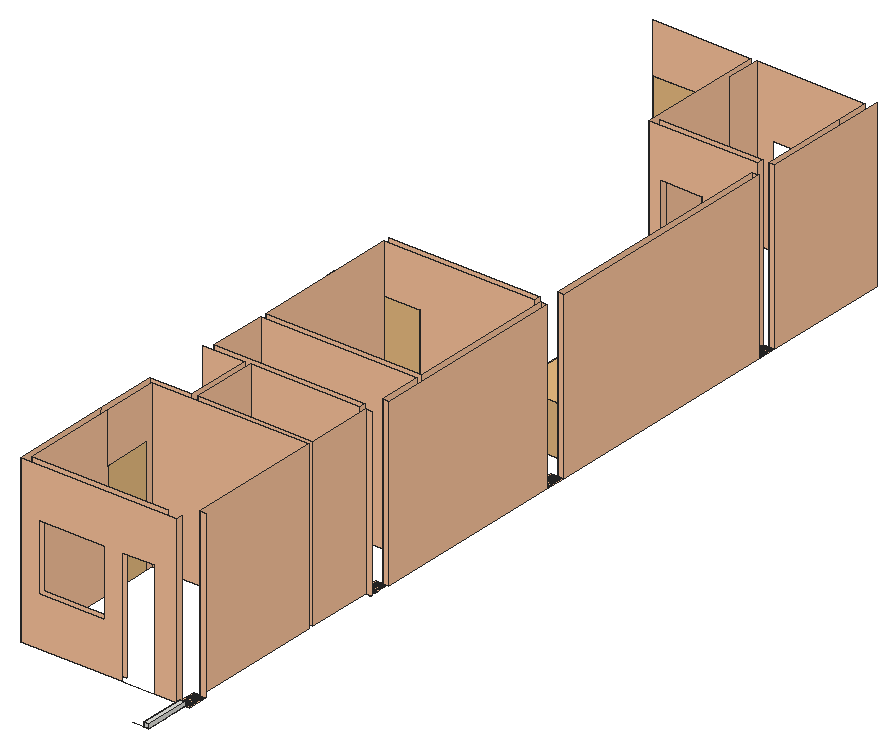
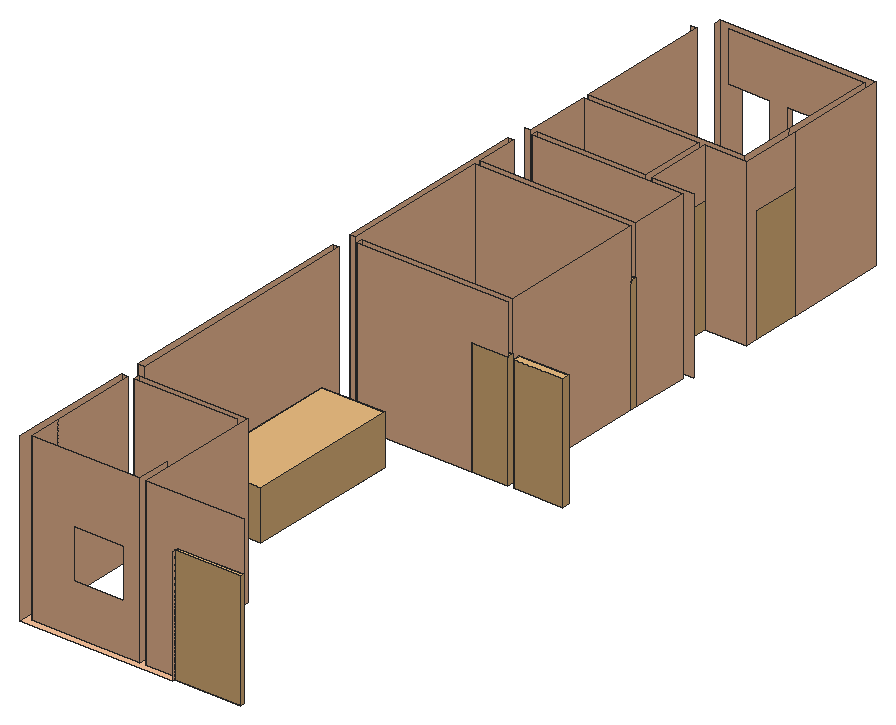
# SketchUp Ruby script. Lengths in inches.
U = 1.inch
M = Sketchup.active_model
def pt(a) = Geom::Point3d.new(a.map { |v| v * U })
def face(e, loops, mat)
  f = e.add_face(loops[0].map { |a| pt(a) })
  loops[1..].each { |l| e.add_face(l.map { |a| pt(a) }).erase! }
  f.material = f.back_material = mat if mat
  f
end
# faces: each face lists its corners as indices into pts; further lists are holes
def faces(e, pts, list, mat = nil) = list.each { |f| face(e, (f[0].is_a?(Array) ? f : [f]).map { |l| l.map { |i| pts[i] } }, mat) }
# xy, xz, yz: faces in a plane at the given z, y or x. An outline is a flat list of corners, or four numbers for a rectangle; further outlines are holes
def ring(l) = l.size == 4 ? [[l[0], l[1]], [l[2], l[1]], [l[2], l[3]], [l[0], l[3]]] : l.each_slice(2).to_a
def flat(e, list, mat, &to3) = list.each { |f| face(e, (f[0].is_a?(Array) ? f : [f]).map { |l| ring(l).map { |u, v| to3.(u, v) } }, mat) }
def xy(e, z, list, mat = nil) = flat(e, list, mat) { |x, y| [x, y, z] }
def xz(e, y, list, mat = nil) = flat(e, list, mat) { |x, z| [x, y, z] }
def yz(e, x, list, mat = nil) = flat(e, list, mat) { |y, z| [x, y, z] }
def lines(e, pts, list) = list.each { |a, b| e.add_line(pt(pts[a]), pt(pts[b])) }
# prism: a flat outline (further loops are holes) pulled along v
def prism(e, loops, v, mat = nil)
  f = face(e, loops, mat); d = Geom::Vector3d.new(v.map { |x| x * U })
  f.pushpull(f.normal.samedirection?(d) ? d.length : -d.length)
end
def box(e, o, s, mat = nil) = prism(e, [[o, [o[0] + s[0], o[1], o[2]], [o[0] + s[0], o[1] + s[1], o[2]], [o[0], o[1] + s[1], o[2]]]], [0, 0, s[2]], mat)
def at(x, y, z, deg = 0) = Geom::Transformation.translation(pt([x, y, z])) * Geom::Transformation.rotation(ORIGIN, Z_AXIS, deg.degrees)
def axes(o, x, y, z) = Geom::Transformation.new([*x, 0, *y, 0, *z, 0, *pt(o).to_a, 1])
def part(name) = M.definitions.add(name)
# library, detail: a bought-in or finely detailed component or shape, given as its bounding box
def library(name, o, s) = part(name).tap { |d| box(d.entities, o, s) }
def detail(e, o, s) = box(e.add_group.entities, o, s)
def put(e, d, t, mat = nil) = e.add_instance(d, t).tap { |i| i.material = mat if mat }
def group(e, t, mat = nil) = e.add_group.tap { |g| g.transformation = t; g.material = mat if mat }.entities
root = M.entities
M.materials.add("[Color A01]2").color = [255, 204, 204]
M.materials.add("[Color A02]1").color = [252, 197, 157]
c1 = library("Group\#55",[0,0,0],[42.67,2.97,87.375])
c2 = library("Group\#37",[0,0,0],[42.67,2.97,87.375])
c3 = library("Group\#46",[0,0,0],[42.67,2.97,87.375])
c4 = library("Sliding door\#1",[32.62,66.51,0],[146.81,8.35,98.97])
c5 = library("Sofa 005",[-44.88,-17.99,0],[89.76,35.98,35.98])
box(root,[168.96,13.0625,131.89],[3.93,33,3])
xy(root,131.89,[[150.53,46.0625,166.9,50.62],[166.9,46.0625,175.89,46.0625,175.89,61,171.33,61,171.33,60.12,174.88,60.12,174.88,47.08,167.91,47.08,167.91,50.62,166.9,50.62],[167.91,47.08,168.17,47.08,168.54,47.46,167.91,48.09],[168.17,47.08,168.93,47.08,168.54,47.46],[168.93,47.08,169.94,47.08,170.32,47.46,169.42,48.35,168.54,47.46],
  [169.94,47.08,170.7,47.08,170.32,47.46],[170.7,47.08,171.71,47.08,172.09,47.46,171.19,48.36,170.32,47.46],[171.71,47.08,172.47,47.08,172.09,47.46],[172.47,47.08,173.49,47.08,173.85,47.47,172.95,48.37,172.09,47.46],[173.49,47.08,174.25,47.08,173.85,47.47],
  [174.25,47.08,174.88,47.08,174.88,48.22,174.7,48.4,173.85,47.47],[168.54,47.46,169.42,48.35,168.54,49.23,167.91,48.6,167.91,48.09],[170.32,47.46,171.19,48.36,170.3,49.25,169.42,48.35],[172.09,47.46,172.95,48.37,172.07,49.26,171.19,48.36],[173.85,47.47,174.7,48.4,173.82,49.27,172.95,48.37],
  [174.88,48.22,174.88,48.6,174.7,48.4],[169.42,48.35,170.3,49.25,169.42,50.13,168.54,49.23],[171.19,48.36,172.07,49.26,171.18,50.14,170.3,49.25],[172.95,48.37,173.82,49.27,172.94,50.15,172.07,49.26],[174.7,48.4,174.88,48.6,174.88,49.99,174.69,50.17,173.82,49.27],
  [167.91,48.6,168.54,49.23,167.91,49.86],[168.54,49.23,169.42,50.13,168.93,50.62,168.16,50.62,167.91,50.37,167.91,49.86],[170.3,49.25,171.18,50.14,170.7,50.62,169.9,50.62,169.42,50.13],[172.07,49.26,172.94,50.15,172.06,51.04,171.18,50.14],[173.82,49.27,174.69,50.17,173.82,51.05,172.94,50.15],
  [174.88,49.99,174.88,50.37,174.69,50.17],[169.42,50.13,169.9,50.62,168.93,50.62],[171.18,50.14,172.06,51.04,171.33,51.76,171.33,50.62,170.7,50.62],[172.94,50.15,173.82,51.05,172.93,51.93,172.06,51.04],[174.69,50.17,174.88,50.37,174.88,51.76,174.69,51.95,173.82,51.05],
  [167.91,50.37,168.16,50.62,167.91,50.62],[166.9,50.62,167.91,50.62,167.91,60.12,171.33,60.12,171.33,61.13,166.9,61.13],[167.91,50.62,168.16,50.62,168.54,51.01,167.91,51.63],[168.16,50.62,168.93,50.62,168.54,51.01],[168.93,50.62,169.9,50.62,170.3,51.02,169.42,51.9,168.54,51.01],
  [169.9,50.62,170.7,50.62,170.3,51.02],[170.7,50.62,171.33,50.62,171.33,51.76,171.18,51.92,170.3,51.02],[168.54,51.01,169.42,51.9,168.54,52.78,167.91,52.14,167.91,51.63],[170.3,51.02,171.18,51.92,170.3,52.8,169.42,51.9],[172.06,51.04,172.93,51.93,172.06,52.8125,171.33,52.08,171.33,51.76],
  [173.82,51.05,174.69,51.95,173.8125,52.83,172.93,51.93],[171.33,51.76,171.33,52.08,171.18,51.92],[174.88,51.76,174.88,52.14,174.69,51.95],[169.42,51.9,170.3,52.8,169.42,53.67,168.54,52.78],[171.18,51.92,171.33,52.08,171.33,53.53,171.18,53.69,170.3,52.8],
  [172.93,51.93,173.8125,52.83,172.93,53.71,172.06,52.8125],[174.69,51.95,174.88,52.14,174.88,53.53,174.69,53.72,173.8125,52.83],[171.33,52.08,172.06,52.8125,171.33,53.53],[167.91,52.14,168.54,52.78,167.91,53.41],[168.54,52.78,169.42,53.67,168.55,54.55,167.91,53.91,167.91,53.41],
  [170.3,52.8,171.18,53.69,170.3,54.57,169.42,53.67],[172.06,52.8125,172.93,53.71,172.06,54.58,171.33,53.85,171.33,53.53],[173.8125,52.83,174.69,53.72,173.8125,54.6,172.93,53.71],[171.33,53.53,171.33,53.85,171.18,53.69],[174.88,53.53,174.88,53.91,174.69,53.72],
  [169.42,53.67,170.3,54.57,169.43,55.43,168.55,54.55],[171.18,53.69,171.33,53.85,171.33,55.31,171.18,55.46,170.3,54.57],[172.93,53.71,173.8125,54.6,172.93,55.48,172.06,54.58],[171.33,53.85,172.06,54.58,171.33,55.31],[167.91,53.91,168.55,54.55,167.91,55.18],
  [168.55,54.55,169.43,55.43,168.55,56.32,167.91,55.6875,167.91,55.18],[170.3,54.57,171.18,55.46,170.32,56.32,169.43,55.43],[172.06,54.58,172.93,55.48,172.06,56.36,171.33,55.62,171.33,55.31],[173.8125,54.6,174.69,55.49,173.8125,56.37,172.93,55.48],[171.33,55.31,171.33,55.62,171.18,55.46],
  [169.43,55.43,170.32,56.32,169.43,57.21,168.55,56.32],[171.18,55.46,171.33,55.62,171.33,57.08,171.21,57.21,170.32,56.32],[172.93,55.48,173.8125,56.37,172.93,57.25,172.06,56.36],[174.69,55.49,174.88,55.6875,174.88,57.08,174.69,57.27,173.8125,56.37],[171.33,55.62,172.06,56.36,171.33,57.08],
  [167.91,55.6875,168.55,56.32,167.91,56.95],[168.55,56.32,169.43,57.21,168.55,58.09,167.91,57.46,167.91,56.95],[170.32,56.32,171.21,57.21,170.32,58.09,169.43,57.21],[172.06,56.36,172.93,57.25,172.09,58.09,171.33,57.33,171.33,57.08],[173.8125,56.37,174.69,57.27,173.8125,58.15,172.93,57.25],
  [171.33,57.08,171.33,57.33,171.21,57.21],[174.88,57.08,174.88,57.46,174.69,57.27],[169.43,57.21,170.32,58.09,169.43,58.98,168.55,58.09],[171.21,57.21,171.33,57.33,171.33,58.85,171.21,58.98,170.32,58.09],[172.93,57.25,173.8125,58.15,172.98,58.98,172.09,58.09],
  [174.69,57.27,174.88,57.46,174.88,58.85,174.69,59.04,173.8125,58.15],[171.33,57.33,172.09,58.09,171.33,58.85],[168.55,58.09,169.43,58.98,168.55,59.86,167.91,59.23,167.91,58.73],[170.32,58.09,171.21,58.98,170.32,59.86,169.43,58.98],[172.09,58.09,172.98,58.98,172.09,59.86,171.33,59.11,171.33,58.85],
  [173.8125,58.15,174.69,59.04,173.87,59.86,172.98,58.98],[171.33,58.85,171.33,59.11,171.21,58.98],[174.88,58.85,174.88,59.23,174.69,59.04],[169.43,58.98,170.32,59.86,170.07,60.12,168.8,60.12,168.55,59.86],[171.21,58.98,171.33,59.11,171.33,60.12,170.57,60.12,170.32,59.86],
  [172.98,58.98,173.87,59.86,173.61,60.12,172.35,60.12,172.09,59.86],[174.69,59.04,174.88,59.23,174.88,60.12,174.12,60.12,173.87,59.86],[171.33,59.11,172.09,59.86,171.84,60.12,171.33,60.12],[167.91,59.23,168.55,59.86,168.29,60.12,167.91,60.12],[168.55,59.86,168.8,60.12,168.29,60.12],
  [170.32,59.86,170.57,60.12,170.07,60.12],[172.09,59.86,172.35,60.12,171.84,60.12],[173.87,59.86,174.12,60.12,173.61,60.12],[166.89,212.2,166.9,216.63],[171.33,212.2,175.89,212.21],
  [167.91,213.21,168.17,213.21,168.55,213.59,167.91,214.22],[168.93,213.21,169.94,213.21,170.32,213.59,169.43,214.48,168.55,213.59],[169.94,213.21,170.7,213.21,170.32,213.59],[170.7,213.21,171.71,213.21,172.09,213.59,171.21,214.48,170.32,213.59],[171.71,213.21,172.47,213.21,172.09,213.59],
  [172.47,213.21,173.49,213.21,173.87,213.59,172.98,214.48,172.09,213.59],[173.49,213.21,174.25,213.21,173.87,213.59],[174.25,213.21,174.88,213.21,174.88,214.22,174.69,214.42,173.87,213.59],[168.55,213.59,169.43,214.48,168.55,215.36,167.91,214.73,167.91,214.22],[170.32,213.59,171.21,214.48,170.32,215.36,169.43,214.48],
  [172.09,213.59,172.98,214.48,172.09,215.36,171.21,214.48],[173.87,213.59,174.69,214.42,173.8125,215.3125,172.98,214.48],[169.43,214.48,170.32,215.36,169.43,216.25,168.55,215.36],[171.21,214.48,172.09,215.36,171.21,216.25,170.32,215.36],[172.98,214.48,173.8125,215.3125,172.93,216.21,172.09,215.36],
  [167.91,214.73,168.55,215.36,167.91,216],[173.8125,215.3125,174.69,216.1875,173.8125,217.08,172.93,216.21],[168.55,215.36,169.43,216.25,169.05,216.63,168.04,216.63,167.91,216.5,167.91,216],[170.32,215.36,171.21,216.25,170.83,216.63,169.8125,216.63,169.43,216.25],[172.09,215.36,172.93,216.21,172.06,217.1,171.21,216.25],
  [174.88,216,174.88,216.38,174.69,216.1875],[174.69,216.1875,174.88,216.38,174.88,217.77,174.6875,217.96,173.8125,217.08],[172.93,216.21,173.8125,217.08,172.93,217.98,172.06,217.1],[169.43,216.25,169.8125,216.63,169.05,216.63],[171.21,216.25,172.06,217.1,171.33,217.83,171.33,216.63,170.83,216.63],
  [167.91,216.5,168.04,216.63,167.91,216.63],[166.9,216.63,167.91,216.63,167.91,226.13,171.33,226.13,171.33,227.14,166.9,227.14],[167.91,216.63,168.04,216.63,168.55,217.14,167.91,217.77],[169.05,216.63,169.8125,216.63,170.32,217.14,169.43,218.02,168.55,217.14],[169.8125,216.63,170.83,216.63,170.32,217.14],
  [170.83,216.63,171.33,216.63,171.33,217.83,171.18,217.99,170.32,217.14],[173.8125,217.08,174.6875,217.96,173.8,218.85,172.93,217.98],[172.06,217.1,172.93,217.98,172.06,218.87,171.33,218.15,171.33,217.83],[168.55,217.14,169.43,218.02,168.55,218.91,167.91,218.28,167.91,217.77],[170.32,217.14,171.18,217.99,170.3,218.89,169.43,218.02],
  [174.88,217.77,174.88,218.15,174.6875,217.96],[171.33,217.83,171.33,218.15,171.18,217.99],[174.6875,217.96,174.88,218.15,174.88,219.54,174.6875,219.73,173.8,218.85],[172.93,217.98,173.8,218.85,172.92,219.73,172.06,218.87],[171.18,217.99,171.33,218.15,171.33,219.61,171.18,219.77,170.3,218.89],
  [171.33,218.15,172.06,218.87,171.33,219.61],[167.91,218.28,168.55,218.91,167.91,219.54],[173.8,218.85,174.6875,219.73,173.8,220.62,172.92,219.73],[172.06,218.87,172.92,219.73,172.03,220.62,171.33,219.92,171.33,219.61],[170.3,218.89,171.18,219.77,170.3,220.66,169.42,219.78],
  [174.88,219.54,174.88,219.92,174.6875,219.73],[171.33,219.61,171.33,219.92,171.18,219.77],[174.6875,219.73,174.88,219.92,174.88,221.32,174.6875,221.51,173.8,220.62],[171.18,219.77,171.33,219.92,171.33,221.32,171.14,221.51,170.3,220.66],[171.33,219.92,172.03,220.62,171.33,221.32],
  [172.03,220.62,172.92,221.51,172.03,222.39,171.33,221.7,171.33,221.32],[173.8,220.62,174.6875,221.51,173.8,222.39,172.92,221.51],[170.3,220.66,171.14,221.51,170.28,222.37,169.44,221.54],[171.33,221.32,171.33,221.7,171.14,221.51],[174.88,221.32,174.88,221.7,174.6875,221.51],
  [171.14,221.51,171.33,221.7,171.33,223.09,171.18,223.25,170.28,222.37],[172.92,221.51,173.8,222.39,172.92,223.28,172.03,222.39],[174.6875,221.51,174.88,221.7,174.88,223.09,174.6875,223.28,173.8,222.39],[169.44,221.54,170.28,222.37,169.39,223.26,168.55,222.44],[171.33,221.7,172.03,222.39,171.33,223.09],
  [167.91,221.82,168.55,222.44,167.91,223.09],[173.8,222.39,174.6875,223.28,173.8,224.16,172.92,223.28],[171.33,223.09,171.33,223.4,171.18,223.25],[174.88,223.09,174.88,223.47,174.6875,223.28],[171.18,223.25,171.33,223.4,171.33,224.86,171.19,225,170.29,224.13],
  [169.39,223.26,170.29,224.13,169.41,225.02,168.5,224.15],[172.92,223.28,173.8,224.16,172.97,225,172.07,224.12],[174.6875,223.28,174.88,223.47,174.88,224.86,174.6875,225.05,173.8,224.16],[167.91,223.6,168.5,224.15,167.91,224.73],[172.07,224.12,172.97,225,172.09,225.88,171.33,225.14,171.33,224.86],
  [168.5,224.15,169.41,225.02,168.53,225.89,167.91,225.37,167.91,224.73],[173.8,224.16,174.6875,225.05,173.86,225.875,172.97,225],[171.33,224.86,171.33,225.14,171.19,225],[174.88,224.86,174.88,225.24,174.6875,225.05],[171.19,225,171.33,225.14,171.33,226.13,170.57,226.13,170.3125,225.88],
  [169.41,225.02,170.3125,225.88,170.07,226.13,168.8,226.13,168.53,225.89],[173.86,225.875,174.12,226.13,173.61,226.13],[170.3125,225.88,170.57,226.13,170.07,226.13],[172.09,225.88,172.35,226.13,171.84,226.13],[168.53,225.89,168.8,226.13,168.29,226.13],
  [171.33,227.14,171.33,258.67,77.375,258.67,77.375,263.23,171.33,263.23,171.33,371.25,175.89,371.25,175.89,227.14],[83.33,371.24,166.9,375.68],[166.9,371.24,171.33,371.24,171.33,371.25,175.89,371.25,175.89,386.1875,171.33,386.1875,171.33,385.3,174.88,385.3,174.88,372.26,167.91,372.26,167.91,375.68,166.9,375.68],[167.91,372.26,168.17,372.26,168.55,372.64,167.91,373.27],[168.17,372.26,168.93,372.26,168.55,372.64],
  [168.93,372.26,169.94,372.26,170.32,372.64,169.43,373.52,168.55,372.64],[169.94,372.26,170.7,372.26,170.32,372.64],[170.7,372.26,171.71,372.26,172.09,372.64,171.21,373.52,170.32,372.64],[171.71,372.26,172.47,372.26,172.09,372.64],[172.47,372.26,173.49,372.26,173.87,372.64,172.98,373.52,172.09,372.64],
  [173.49,372.26,174.25,372.26,173.87,372.64],[174.25,372.26,174.88,372.26,174.88,373.27,174.69,373.46,173.87,372.64],[168.55,372.64,169.43,373.52,168.55,374.41,167.91,373.78,167.91,373.27],[170.32,372.64,171.21,373.52,170.32,374.41,169.43,373.52],[172.09,372.64,172.98,373.52,172.09,374.41,171.21,373.52],
  [173.87,372.64,174.69,373.46,173.8125,374.36,172.98,373.52],[174.88,373.27,174.88,373.65,174.69,373.46],[174.69,373.46,174.88,373.65,174.88,375.04,174.69,375.23,173.8125,374.36],[169.43,373.52,170.32,374.41,169.43,375.3,168.55,374.41],[171.21,373.52,172.09,374.41,171.21,375.3,170.32,374.41],
  [172.98,373.52,173.8125,374.36,172.93,375.25,172.09,374.41],[167.91,373.78,168.55,374.41,167.91,375.04],[173.8125,374.36,174.69,375.23,173.8125,376.13,172.93,375.25],[168.55,374.41,169.43,375.3,169.05,375.68,168.04,375.68,167.91,375.55,167.91,375.04],[170.32,374.41,171.21,375.3,170.83,375.68,169.8125,375.68,169.43,375.3],
  [172.09,374.41,172.93,375.25,172.06,376.14,171.21,375.3],[174.88,375.04,174.88,375.42,174.69,375.23],[174.69,375.23,174.88,375.42,174.88,376.82,174.69,377.01,173.8125,376.13],[172.93,375.25,173.8125,376.13,172.93,377.02,172.06,376.14],[169.43,375.3,169.8125,375.68,169.05,375.68],
  [171.21,375.3,172.06,376.14,171.33,376.88,171.33,375.68,170.83,375.68],[167.91,375.55,168.04,375.68,167.91,375.68],[166.9,375.68,167.91,375.68,167.91,385.3,171.33,385.3,171.33,386.1875,166.9,386.1875],[167.91,375.68,168.04,375.68,168.55,376.18,167.91,376.82],[168.04,375.68,169.05,375.68,168.55,376.18],
  [169.05,375.68,169.8125,375.68,170.32,376.18,169.43,377.07,168.55,376.18],[169.8125,375.68,170.83,375.68,170.32,376.18],[170.83,375.68,171.33,375.68,171.33,376.88,171.18,377.04,170.32,376.18],[173.8125,376.13,174.69,377.01,173.8125,377.9,172.93,377.02],[172.06,376.14,172.93,377.02,172.06,377.92,171.33,377.19,171.33,376.88],
  [168.55,376.18,169.43,377.07,168.55,377.95,167.91,377.32,167.91,376.82],[170.32,376.18,171.18,377.04,170.3,377.93,169.43,377.07],[174.88,376.82,174.88,377.19,174.69,377.01],[171.33,376.88,171.33,377.19,171.18,377.04],[174.69,377.01,174.88,377.19,174.88,378.59,174.69,378.78,173.8125,377.9],
  [172.93,377.02,173.8125,377.9,172.93,378.8,172.06,377.92],[171.18,377.04,171.33,377.19,171.33,378.65,171.18,378.8125,170.3,377.93],[169.43,377.07,170.3,377.93,169.42,378.83,168.55,377.95],[171.33,377.19,172.06,377.92,171.33,378.65],[167.91,377.32,168.55,377.95,167.91,378.59],
  [173.8125,377.9,174.69,378.78,173.8125,379.67,172.93,378.8],[172.06,377.92,172.93,378.8,172.06,379.69,171.33,378.97,171.33,378.65],[170.3,377.93,171.18,378.8125,170.3,379.71,169.42,378.83],[168.55,377.95,169.42,378.83,168.54,379.72,167.91,379.09,167.91,378.59],[174.88,378.59,174.88,378.97,174.69,378.78],
  [171.33,378.65,171.33,378.97,171.18,378.8125],[174.69,378.78,174.88,378.97,174.88,380.36,174.69,380.55,173.8125,379.67],[172.93,378.8,173.8125,379.67,172.93,380.57,172.06,379.69],[171.18,378.8125,171.33,378.97,171.33,380.43,171.18,380.58,170.3,379.71],[169.42,378.83,170.3,379.71,169.42,380.6,168.54,379.72],
  [171.33,378.97,172.06,379.69,171.33,380.43],[167.91,379.09,168.54,379.72,167.91,380.36],[173.8125,379.67,174.69,380.55,173.82,381.45,172.93,380.57],[172.06,379.69,172.93,380.57,172.06,381.46,171.33,380.74,171.33,380.43],[170.3,379.71,171.18,380.58,170.3,381.48,169.42,380.6],
  [168.54,379.72,169.42,380.6,168.54,381.49,167.91,380.87,167.91,380.36],[174.88,380.36,174.88,380.74,174.69,380.55],[171.33,380.43,171.33,380.74,171.18,380.58],[174.69,380.55,174.88,380.74,174.88,382.13,174.69,382.33,173.82,381.45],[172.93,380.57,173.82,381.45,172.94,382.35,172.06,381.46],
  [171.18,380.58,171.33,380.74,171.33,382.2,171.18,382.36,170.3,381.48],[169.42,380.6,170.3,381.48,169.42,382.37,168.54,381.49],[171.33,380.74,172.06,381.46,171.33,382.2],[167.91,380.87,168.54,381.49,167.91,382.13],[173.82,381.45,174.69,382.33,173.82,383.23,172.94,382.35],
  [172.06,381.46,172.94,382.35,172.07,383.25,171.33,382.51,171.33,382.2],[170.3,381.48,171.18,382.36,170.3,383.25,169.42,382.37],[168.54,381.49,169.42,382.37,168.54,383.27,167.91,382.64,167.91,382.13],[174.88,382.13,174.88,382.51,174.69,382.33],[171.33,382.2,171.33,382.51,171.18,382.36],
  [174.69,382.33,174.88,382.51,174.88,383.91,174.7,384.11,173.82,383.23],[172.94,382.35,173.82,383.23,172.96,384.14,172.07,383.25],[171.18,382.36,171.33,382.51,171.33,384,171.19,384.14,170.3,383.25],[169.42,382.37,170.3,383.25,169.42,384.15,168.54,383.27],[171.33,382.51,172.07,383.25,171.33,384],
  [167.91,382.64,168.54,383.27,167.91,383.91],[173.82,383.23,174.7,384.11,173.85,385.03,172.96,384.14],[170.3,383.25,171.19,384.14,170.32,385.04,169.42,384.15],[172.07,383.25,172.96,384.14,172.09,385.04,171.33,384.29,171.33,384],[168.54,383.27,169.42,384.15,168.54,385.04,167.91,384.41,167.91,383.91],
  [174.88,383.91,174.88,384.29,174.7,384.11],[171.33,384,171.33,384.29,171.19,384.14],[174.7,384.11,174.88,384.29,174.88,385.3,174.12,385.3,173.85,385.03],[171.19,384.14,171.33,384.29,171.33,385.3,170.57,385.3,170.32,385.04],[172.96,384.14,173.85,385.03,173.61,385.3,172.35,385.3,172.09,385.04],
  [169.42,384.15,170.32,385.04,170.07,385.3,168.8,385.3,168.54,385.04],[171.33,384.29,172.09,385.04,171.84,385.3,171.33,385.3],[167.91,384.41,168.54,385.04,168.29,385.3,167.91,385.3],[173.85,385.03,174.12,385.3,173.61,385.3],[168.54,385.04,168.8,385.3,168.29,385.3],
  [170.32,385.04,170.57,385.3,170.07,385.3],[172.09,385.04,172.35,385.3,171.84,385.3],[166.9,563.34,171.33,563.34,171.33,564.35,167.91,564.35,167.91,573.85,166.9,573.85],[171.33,563.34,175.89,563.34,175.89,578.28,166.9,578.28,166.9,573.85,167.91,573.85,167.91,577.27,174.88,577.27,174.88,564.35,171.33,564.35],[167.91,564.35,168.17,564.35,168.55,564.73,167.91,565.36],
  [168.17,564.35,168.93,564.35,168.55,564.73],[168.93,564.35,169.94,564.35,170.32,564.73,169.43,565.62,168.55,564.73],[169.94,564.35,170.7,564.35,170.32,564.73],[170.7,564.35,171.33,564.35,171.33,565.49,171.21,565.62,170.32,564.73],[171.33,564.35,171.71,564.35,172.09,564.73,171.33,565.49],
  [171.71,564.35,172.47,564.35,172.09,564.73],[172.47,564.35,173.49,564.35,173.87,564.73,172.98,565.62,172.09,564.73],[173.49,564.35,174.25,564.35,173.87,564.73],[174.25,564.35,174.88,564.35,174.88,565.36,174.69,565.56,173.87,564.73],[168.55,564.73,169.43,565.62,168.55,566.5,167.91,565.87,167.91,565.36],
  [170.32,564.73,171.21,565.62,170.32,566.5,169.43,565.62],[172.09,564.73,172.98,565.62,172.09,566.5,171.33,565.74,171.33,565.49],[173.87,564.73,174.69,565.56,173.8125,566.45,172.98,565.62],[174.88,565.36,174.88,565.74,174.69,565.56],[171.33,565.49,171.33,565.74,171.21,565.62],
  [174.69,565.56,174.88,565.74,174.88,567.14,174.6875,567.33,173.8125,566.45],[169.43,565.62,170.32,566.5,169.43,567.39,168.55,566.5],[171.21,565.62,171.33,565.74,171.33,567.26,171.21,567.39,170.32,566.5],[172.98,565.62,173.8125,566.45,172.93,567.34,172.09,566.5],[171.33,565.74,172.09,566.5,171.33,567.26],
  [167.91,565.87,168.55,566.5,167.91,567.14],[173.8125,566.45,174.6875,567.33,173.8,568.21,172.93,567.34],[168.55,566.5,169.43,567.39,168.55,568.28,167.91,567.64,167.91,567.14],[170.32,566.5,171.21,567.39,170.32,568.28,169.43,567.39],[172.09,566.5,172.93,567.34,172.06,568.24,171.33,567.52,171.33,567.26],
  [174.88,567.14,174.88,567.52,174.6875,567.33],[171.33,567.26,171.33,567.52,171.21,567.39],[174.6875,567.33,174.88,567.52,174.88,568.91,174.6875,569.1,173.8,568.21],[172.93,567.34,173.8,568.21,172.92,569.1,172.06,568.24],[169.43,567.39,170.32,568.28,169.43,569.16,168.55,568.28],
  [171.21,567.39,171.33,567.52,171.33,568.97,171.18,569.13,170.32,568.28],[171.33,567.52,172.06,568.24,171.33,568.97],[167.91,567.64,168.55,568.28,167.91,568.91],[173.8,568.21,174.6875,569.1,173.8,569.99,172.92,569.1],[172.06,568.24,172.92,569.1,172.03,569.99,171.33,569.29,171.33,568.97],
  [168.55,568.28,169.43,569.16,168.55,570.05,167.91,569.42,167.91,568.91],[170.32,568.28,171.18,569.13,170.3,570.03,169.43,569.16],[174.88,568.91,174.88,569.29,174.6875,569.1],[171.33,568.97,171.33,569.29,171.18,569.13],[172.92,569.1,173.8,569.99,172.92,570.87,172.03,569.99],
  [174.6875,569.1,174.88,569.29,174.88,570.68,174.6875,570.87,173.8,569.99],[171.18,569.13,171.33,569.29,171.33,570.68,171.14,570.87,170.3,570.03],[169.43,569.16,170.3,570.03,169.42,570.92,168.55,570.05],[171.33,569.29,172.03,569.99,171.33,570.68],[167.91,569.42,168.55,570.05,167.91,570.68],
  [172.03,569.99,172.92,570.87,172.03,571.76,171.33,571.0625,171.33,570.68],[173.8,569.99,174.6875,570.87,173.8,571.76,172.92,570.87],[170.3,570.03,171.14,570.87,170.26,571.76,169.42,570.92],[168.55,570.05,169.42,570.92,168.55,571.81,167.91,571.1875,167.91,570.68],[171.33,570.68,171.33,571.0625,171.14,570.87],
  [174.88,570.68,174.88,571.0625,174.6875,570.87],[171.14,570.87,171.33,571.0625,171.33,572.46,171.14,572.65,170.26,571.76],[172.92,570.87,173.8,571.76,172.92,572.65,172.03,571.76],[174.6875,570.87,174.88,571.0625,174.88,572.46,174.6875,572.65,173.8,571.76],[169.42,570.92,170.26,571.76,169.39,572.63,168.55,571.81],
  [171.33,571.0625,172.03,571.76,171.33,572.46],[167.91,571.1875,168.55,571.81,167.91,572.46],[170.26,571.76,171.14,572.65,170.28,573.51,169.39,572.63],[172.03,571.76,172.92,572.65,172.03,573.53,171.33,572.84,171.33,572.46],[173.8,571.76,174.6875,572.65,173.8,573.53,172.92,572.65],
  [168.55,571.81,169.39,572.63,168.49,573.52,167.91,572.96,167.91,572.46],[171.33,572.46,171.33,572.84,171.14,572.65],[174.88,572.46,174.88,572.84,174.6875,572.65],[169.39,572.63,170.28,573.51,169.94,573.85,168.83,573.85,168.49,573.52],[171.14,572.65,171.33,572.84,171.33,573.85,170.63,573.85,170.28,573.51],
  [172.92,572.65,173.8,573.53,172.92,574.42,172.03,573.53],[174.6875,572.65,174.88,572.84,174.88,574.23,174.6875,574.42,173.8,573.53],[171.33,572.84,172.03,573.53,171.18,574.38,170.63,573.85,171.33,573.85],[167.91,572.96,168.49,573.52,168.17,573.85,167.91,573.85],[170.28,573.51,170.63,573.85,169.94,573.85],
  [168.49,573.52,168.83,573.85,168.17,573.85],[172.03,573.53,172.92,574.42,172.07,575.26,171.18,574.38],[173.8,573.53,174.6875,574.42,173.8,575.3,172.92,574.42],[87.89,573.85,87.89,665.91,64.84,665.91,64.84,670.34,175.89,670.34,175.89,578.28,171.33,578.28,171.33,665.91,92.44,665.91,92.44,578.28,96.37,578.28,96.37,573.85],[126.38,573.85,166.9,578.28],
  [167.91,573.85,168.17,573.85,167.91,574.1],[168.17,573.85,168.83,573.85,169.39,574.4,168.5,575.29,167.91,574.73,167.91,574.1],[168.83,573.85,169.94,573.85,169.39,574.4],[169.94,573.85,170.63,573.85,171.18,574.38,170.29,575.27,169.39,574.4],[174.88,574.23,174.88,574.61,174.6875,574.42],
  [171.18,574.38,172.07,575.26,171.19,576.14,170.29,575.27],[169.39,574.4,170.29,575.27,169.41,576.16,168.5,575.29],[172.92,574.42,173.8,575.3,172.97,576.14,172.07,575.26],[174.6875,574.42,174.88,574.61,174.88,576,174.6875,576.19,173.8,575.3],[167.91,574.73,168.5,575.29,167.91,575.875],
  [172.07,575.26,172.97,576.14,172.09,577.02,171.19,576.14],[170.29,575.27,171.19,576.14,170.3125,577.02,169.41,576.16],[168.5,575.29,169.41,576.16,168.53,577.03,167.91,576.51,167.91,575.875],[173.8,575.3,174.6875,576.19,173.86,577.02,172.97,576.14],[174.88,576,174.88,576.38,174.6875,576.19],
  [171.19,576.14,172.09,577.02,171.84,577.27,170.57,577.27,170.3125,577.02],[172.97,576.14,173.86,577.02,173.61,577.27,172.35,577.27,172.09,577.02],[169.41,576.16,170.3125,577.02,170.07,577.27,168.8,577.27,168.53,577.03],[174.6875,576.19,174.88,576.38,174.88,577.27,174.12,577.27,173.86,577.02],[167.91,576.51,168.53,577.03,168.29,577.27,167.91,577.27],
  [170.3125,577.02,170.57,577.27,170.07,577.27],[172.09,577.02,172.35,577.27,171.84,577.27],[173.86,577.02,174.12,577.27,173.61,577.27],[168.53,577.03,168.8,577.27,168.29,577.27]],"[Color A02]1")
xz(root,46.0625,[[[52.9375,131.89,126.53,131.89,126.53,215.89,150.53,215.89,150.53,131.89,166.9,131.89,166.9,251.89,52.9375,251.89],[66.6875,167.89,114.6875,215.89]]],"[Color A02]1")
xz(root,50.62,[[[57.37,131.89,57.37,251.89,156.53,251.89,156.53,215.89,126.53,215.89,126.53,131.89],[66.6875,167.89,114.6875,215.89]]],"[Color A02]1")
xz(root,61,[[171.33,131.89,175.89,251.89]],"[Color A02]1")
xz(root,119.63,[[52.9375,131.89,57.37,215.89]],"[Color A02]1")
xz(root,160.15,[[57.37,131.89,171.33,251.89]],"[Color A02]1")
xz(root,164.21,[[52.9375,131.89,82.95,251.89],[82.95,131.89,82.95,215.89,87.38,215.89,87.38,251.89,171.33,251.89,171.33,131.89]],"[Color A02]1")
xz(root,212.2,[[52.9375,131.89,82.95,251.89],[87.38,131.89,166.89,251.89]],"[Color A02]1")
xz(root,212.21,[[171.33,131.89,175.89,251.89]],"[Color A02]1")
xz(root,216.63,[[57.37,131.89,166.89,251.89]],"[Color A02]1")
xz(root,227.14,[[171.33,131.89,175.89,251.89]],"[Color A02]1")
xz(root,258.67,[[77.375,131.89,171.33,131.89,171.33,251.89,57.37,251.89,57.37,215.89,77.375,215.89]],"[Color A02]1")
xz(root,263.23,[[77.375,131.89,77.375,215.89,57.37,215.89,57.37,251.89,171.33,251.89,171.33,131.89]],"[Color A02]1")
xz(root,371.24,[[83.33,131.89,166.9,131.89,166.9,251.89,57.37,251.89,57.37,215.89,83.33,215.89]],"[Color A02]1")
xz(root,371.25,[[171.33,131.89,175.89,251.89]],"[Color A02]1")
xz(root,375.68,[[83.33,131.89,83.33,215.89,57.37,215.89,57.37,251.89,166.9,251.89,166.9,131.89]],"[Color A02]1")
xz(root,386.1875,[[171.33,131.89,175.89,251.89]],"[Color A02]1")
xz(root,563.34,[[171.33,131.89,175.89,251.89]],"[Color A02]1")
xz(root,573.85,[[87.89,131.89,96.37,131.89,96.37,215.89,126.38,215.89,126.38,131.89,166.9,131.89,166.9,251.89,87.89,251.89]],"[Color A02]1")
xz(root,578.28,[[92.44,131.89,92.44,251.89,166.9,251.89,166.9,131.89,126.38,131.89,126.38,215.89,96.37,215.89,96.37,131.89],[171.33,131.89,175.89,251.89]],"[Color A02]1")
xz(root,665.91,[[64.84,131.89,87.89,131.89,87.89,251.89,16.86,251.89,16.86,215.89,64.84,215.89],[[92.44,131.89,171.33,251.89],[104.48,167.89,140.48,203.89]]],"[Color A02]1")
yz(root,52.9375,[[46.0625,131.89,119.63,251.89],[155.6,131.89,155.6,215.89,119.63,215.89,119.63,251.89,164.21,251.89,164.21,131.89]],"[Color A02]1")
yz(root,57.37,[[50.62,131.89,119.63,251.89],[155.6,131.89,160.15,131.89,160.15,251.89,119.63,251.89,119.63,215.89,155.6,215.89],[216.63,131.89,263.23,131.89,263.23,215.89,258.67,215.89,258.67,251.89,216.63,251.89],[263.23,131.89,375.68,131.89,375.68,215.89,371.24,215.89,371.24,251.89,263.23,251.89]],"[Color A02]1")
yz(root,64.84,[[665.91,131.89,670.34,215.89]],"[Color A02]1")
yz(root,77.375,[[258.67,131.89,263.23,215.89]],"[Color A02]1")
yz(root,82.95,[[194.22,131.89,194.22,215.89,164.21,215.89,164.21,251.89,212.2,251.89,212.2,131.89]],"[Color A02]1")
yz(root,83.33,[[371.24,131.89,375.68,215.89]],"[Color A02]1")
yz(root,87.38,[[194.22,131.89,212.2,131.89,212.2,251.89,164.21,251.89,164.21,215.89,194.22,215.89]],"[Color A02]1")
yz(root,87.89,[[573.85,131.89,665.91,251.89]],"[Color A02]1")
yz(root,92.44,[[641.85,131.89,665.91,251.89]],"[Color A02]1")
yz(root,96.37,[[573.85,131.89,578.28,215.89]],"[Color A02]1")
yz(root,126.38,[[573.85,131.89,578.28,215.89]],"[Color A02]1")
yz(root,166.89,[[212.2,131.89,216.63,251.89]],"[Color A02]1")
yz(root,166.9,[[46.0625,131.89,50.62,251.89],[371.24,131.89,375.68,251.89],[573.85,131.89,578.28,251.89]],"[Color A02]1")
yz(root,171.33,[[61,131.89,160.15,251.89],[164.21,131.89,212.21,251.89],[227.14,131.89,258.67,251.89],[263.23,131.89,371.25,251.89],[386.1875,131.89,563.34,251.89],
  [578.28,131.89,641.85,251.89],[641.85,131.89,665.91,251.89]],"[Color A02]1")
yz(root,175.89,[[227.14,131.89,371.25,251.89],[386.1875,131.89,563.34,251.89],[578.28,131.89,670.34,251.89]],"[Color A02]1")
p = [[16.86,61,131.89],[16.86,46.0625,131.89],[172.89,13.0625,131.89],[172.89,46.0625,131.89],[161.03,46.0625,131.89],[161.03,13.0625,131.89],
  [166.9,212.2,131.89],[171.33,212.2,131.89],[126.53,46.0625,131.89],[150.53,46.0625,131.89]]
lines(root,p,[[0,1],[2,3],[3,4],[5,2],[6,7],[8,9]])
put(root,c1,axes([64.84,665.91,131.68],[-1.12463,0,0],[0,0.8968,0],[0,0,0.9637]))
put(root,c2,axes([52.9375,155.6,131.89],[0,-0.84151,0],[1.47,0,0],[0,0,0.96138]))
put(root,c1,axes([83.33,375.68,131.89],[-0.60843,0,0],[0,-1.47,0],[0,0,0.96138]))
put(root,c3,axes([82.95,194.22,131.89],[0,-0.7034,0],[1.47,0,0],[0,0,0.96138]))
put(root,c1,axes([77.375,263.23,131.89],[-0.46894,0,0],[0,-1.47,0],[0,0,0.96138]))
put(root,c4,axes([8.84,328.55,131.89],[0.24577,0,0],[0,0.6328,0],[0,0,0.8487]))
put(root,c5,axes([148.16,458.79,131.89],[0,-1.25,0],[1.27,0,0],[0,0,1]),"[Color A01]2")
